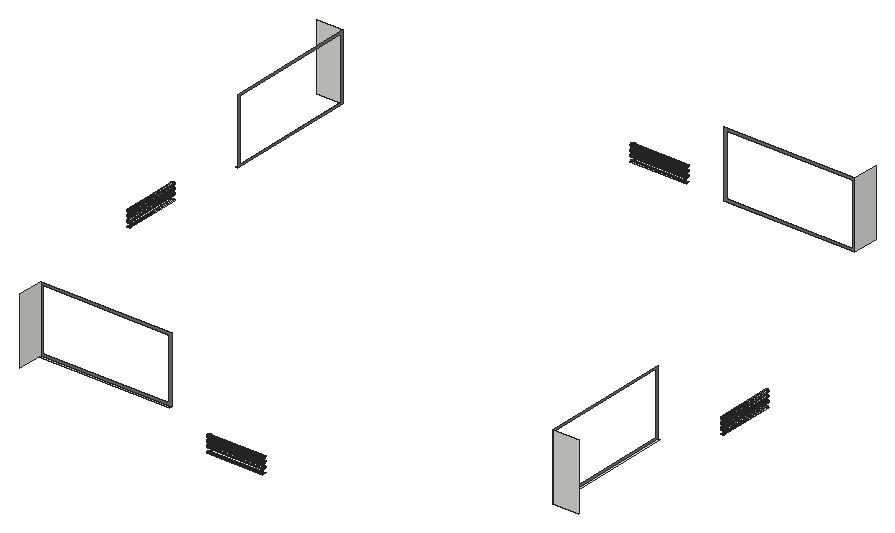
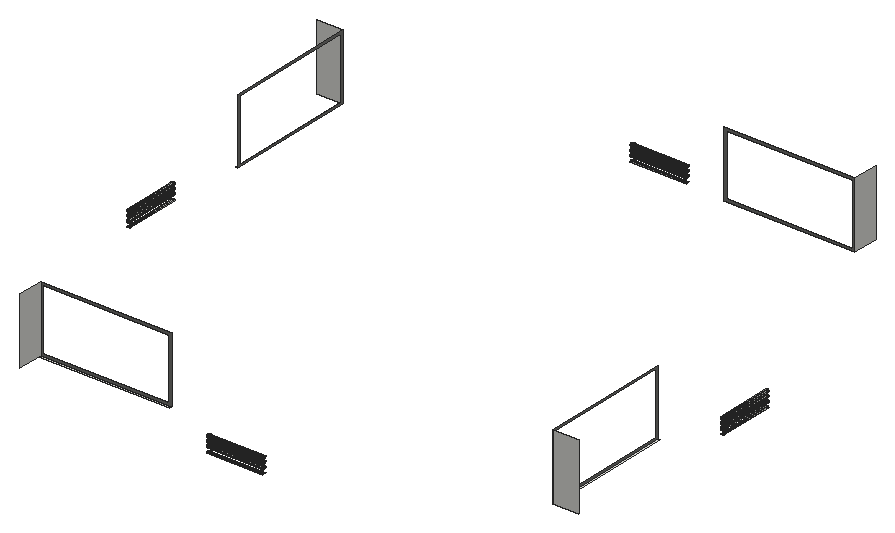
# SketchUp Ruby script. Lengths in inches.
U = 1.inch
M = Sketchup.active_model
def pt(a) = Geom::Point3d.new(a.map { |v| v * U })
def face(e, loops, mat)
  f = e.add_face(loops[0].map { |a| pt(a) })
  loops[1..].each { |l| e.add_face(l.map { |a| pt(a) }).erase! }
  f.material = f.back_material = mat if mat
  f
end
# faces: each face lists its corners as indices into pts; further lists are holes
def faces(e, pts, list, mat = nil) = list.each { |f| face(e, (f[0].is_a?(Array) ? f : [f]).map { |l| l.map { |i| pts[i] } }, mat) }
# xy, xz, yz: faces in a plane at the given z, y or x. An outline is a flat list of corners, or four numbers for a rectangle; further outlines are holes
def ring(l) = l.size == 4 ? [[l[0], l[1]], [l[2], l[1]], [l[2], l[3]], [l[0], l[3]]] : l.each_slice(2).to_a
def flat(e, list, mat, &to3) = list.each { |f| face(e, (f[0].is_a?(Array) ? f : [f]).map { |l| ring(l).map { |u, v| to3.(u, v) } }, mat) }
def xy(e, z, list, mat = nil) = flat(e, list, mat) { |x, y| [x, y, z] }
def xz(e, y, list, mat = nil) = flat(e, list, mat) { |x, z| [x, y, z] }
def yz(e, x, list, mat = nil) = flat(e, list, mat) { |y, z| [x, y, z] }
def lines(e, pts, list) = list.each { |a, b| e.add_line(pt(pts[a]), pt(pts[b])) }
# prism: a flat outline (further loops are holes) pulled along v
def prism(e, loops, v, mat = nil)
  f = face(e, loops, mat); d = Geom::Vector3d.new(v.map { |x| x * U })
  f.pushpull(f.normal.samedirection?(d) ? d.length : -d.length)
end
def box(e, o, s, mat = nil) = prism(e, [[o, [o[0] + s[0], o[1], o[2]], [o[0] + s[0], o[1] + s[1], o[2]], [o[0], o[1] + s[1], o[2]]]], [0, 0, s[2]], mat)
def at(x, y, z, deg = 0) = Geom::Transformation.translation(pt([x, y, z])) * Geom::Transformation.rotation(ORIGIN, Z_AXIS, deg.degrees)
def axes(o, x, y, z) = Geom::Transformation.new([*x, 0, *y, 0, *z, 0, *pt(o).to_a, 1])
def part(name) = M.definitions.add(name)
# library, detail: a bought-in or finely detailed component or shape, given as its bounding box
def library(name, o, s) = part(name).tap { |d| box(d.entities, o, s) }
def detail(e, o, s) = box(e.add_group.entities, o, s)
def put(e, d, t, mat = nil) = e.add_instance(d, t).tap { |i| i.material = mat if mat }
def group(e, t, mat = nil) = e.add_group.tap { |g| g.transformation = t; g.material = mat if mat }.entities
root = M.entities
M.materials.add("[Metal Seamed]").color = [118, 119, 115]
xy(root,533.76,[[306.65,96.8125,641.22,102.8125],[1482,271.47,1488,606.03],[132,943.59,138,1278.16],[978.78,1446.8125,1313.35,1452.8125]])
xz(root,102.8125,[[[306.65,533.76,641.22,702.625],[312.65,539.76,635.22,696.625]]],"[Metal Seamed]")
xz(root,271.47,[[1482,533.76,1548,702.625]])
xz(root,1278.16,[[72,533.76,138,702.625]])
xz(root,1446.8125,[[[978.78,533.76,1313.35,702.625],[984.78,539.76,1307.35,696.625]]],"[Metal Seamed]")
yz(root,138,[[[943.59,533.76,1278.16,702.625],[949.59,539.76,1272.16,696.625]]],"[Metal Seamed]")
yz(root,306.65,[[36.8125,533.76,102.8125,702.625]])
yz(root,1313.35,[[1446.8125,533.76,1512.8125,702.625]])
yz(root,1482,[[[271.47,533.76,606.03,702.625],[277.47,539.76,600.03,696.625]]],"[Metal Seamed]")
p = [[922.01,44.78,502.66],[922.01,45.15,503.55],[778.64,45.15,503.55],[778.64,44.78,502.66],[922.01,51.53,503.55],[922.01,51.9,502.66],
  [778.64,51.9,502.66],[778.64,51.53,503.55],[79.97,662.8,502.66],[80.33,662.8,503.55],[80.33,806.17,503.55],[79.97,806.17,502.66],
  [86.72,662.8,503.55],[87.09,662.8,502.66],[87.09,806.17,502.66],[86.72,806.17,503.55],[1533.28,886.83,503.55],[1532.91,886.83,502.66],
  [1532.91,743.45,502.66],[1533.28,743.45,503.55],[1540.03,886.83,502.66],[1539.67,886.83,503.55],[1539.67,743.45,503.55],[1540.03,743.45,502.66],
  [697.99,1498.09,503.55],[697.99,1497.72,502.66],[841.36,1497.72,502.66],[841.36,1498.09,503.55],[697.99,1504.85,502.66],[697.99,1504.48,503.55],
  [841.36,1504.48,503.55],[841.36,1504.85,502.66],[922.01,45.73,504.3125],[778.64,45.73,504.3125],[922.01,50.95,504.3125],[778.64,50.95,504.3125],
  [80.92,662.8,504.3125],[80.92,806.17,504.3125],[86.13,662.8,504.3125],[86.13,806.17,504.3125],[1533.87,886.83,504.3125],[1533.87,743.45,504.3125],
  [1539.08,886.83,504.3125],[1539.08,743.45,504.3125],[697.99,1498.68,504.3125],[841.36,1498.68,504.3125],[697.99,1503.89,504.3125],[841.36,1503.89,504.3125],
  [922.01,46.5,504.9],[778.64,46.5,504.9],[922.01,50.18,504.9],[778.64,50.18,504.9],[81.68,662.8,504.9],[81.68,806.17,504.9],
  [85.37,662.8,504.9],[85.37,806.17,504.9],[1534.63,886.83,504.9],[1534.63,743.45,504.9],[1538.32,886.83,504.9],[1538.32,743.45,504.9],
  [697.99,1499.44,504.9],[841.36,1499.44,504.9],[697.99,1503.13,504.9],[841.36,1503.13,504.9],[922.01,47.38,505.27],[778.64,47.38,505.27],
  [922.01,49.29,505.27],[778.64,49.29,505.27],[82.57,662.8,505.27],[82.57,806.17,505.27],[84.48,662.8,505.27],[84.48,806.17,505.27],
  [1535.52,886.83,505.27],[1535.52,743.45,505.27],[1537.43,886.83,505.27],[1537.43,743.45,505.27],[697.99,1500.33,505.27],[841.36,1500.33,505.27],
  [697.99,1502.24,505.27],[841.36,1502.24,505.27],[922.01,48.34,505.39],[778.64,48.34,505.39],[83.53,662.8,505.39],[83.53,806.17,505.39],
  [1536.47,886.83,505.39],[1536.47,743.45,505.39],[697.99,1501.28,505.39],[841.36,1501.28,505.39],[922.01,48.34,513.02],[922.01,47.38,513.14],
  [778.64,47.38,513.14],[778.64,48.34,513.02],[922.01,49.29,513.14],[778.64,49.29,513.14],[83.53,662.8,513.02],[82.57,662.8,513.14],
  [82.57,806.17,513.14],[83.53,806.17,513.02],[84.48,662.8,513.14],[84.48,806.17,513.14],[1535.52,886.83,513.14],[1536.47,886.83,513.02],
  [1536.47,743.45,513.02],[1535.52,743.45,513.14],[1537.43,886.83,513.14],[1537.43,743.45,513.14],[697.99,1500.33,513.14],[697.99,1501.28,513.02],
  [841.36,1501.28,513.02],[841.36,1500.33,513.14],[697.99,1502.24,513.14],[841.36,1502.24,513.14],[922.01,46.5,513.51],[778.64,46.5,513.51],
  [922.01,50.18,513.51],[778.64,50.18,513.51],[81.68,662.8,513.51],[81.68,806.17,513.51],[85.37,662.8,513.51],[85.37,806.17,513.51],
  [1534.63,886.83,513.51],[1534.63,743.45,513.51],[1538.32,886.83,513.51],[1538.32,743.45,513.51],[697.99,1499.44,513.51],[841.36,1499.44,513.51],
  [697.99,1503.13,513.51],[841.36,1503.13,513.51],[922.01,45.73,514.1],[778.64,45.73,514.1],[922.01,50.95,514.1],[778.64,50.95,514.1],
  [80.92,662.8,514.1],[80.92,806.17,514.1],[86.13,662.8,514.1],[86.13,806.17,514.1],[1533.87,886.83,514.1],[1533.87,743.45,514.1],
  [1539.08,886.83,514.1],[1539.08,743.45,514.1],[697.99,1498.68,514.1],[841.36,1498.68,514.1],[697.99,1503.89,514.1],[841.36,1503.89,514.1],
  [922.01,45.15,514.86],[778.64,45.15,514.86],[922.01,51.53,514.86],[778.64,51.53,514.86],[80.33,662.8,514.86],[80.33,806.17,514.86],
  [86.72,662.8,514.86],[86.72,806.17,514.86],[1533.28,886.83,514.86],[1533.28,743.45,514.86],[1539.67,886.83,514.86],[1539.67,743.45,514.86],
  [697.99,1498.09,514.86],[841.36,1498.09,514.86],[697.99,1504.48,514.86],[841.36,1504.48,514.86],[922.01,44.78,515.75],[778.64,44.78,515.75],
  [922.01,51.9,515.75],[778.64,51.9,515.75],[79.97,662.8,515.75],[79.97,806.17,515.75],[87.09,662.8,515.75],[87.09,806.17,515.75],
  [1532.91,886.83,515.75],[1532.91,743.45,515.75],[1540.03,886.83,515.75],[1540.03,743.45,515.75],[697.99,1497.72,515.75],[841.36,1497.72,515.75],
  [697.99,1504.85,515.75],[841.36,1504.85,515.75],[922.01,44.65,516.7],[778.64,44.65,516.7],[922.01,52.03,516.7],[778.64,52.03,516.7],
  [79.84,662.8,516.7],[79.84,806.17,516.7],[87.21,662.8,516.7],[87.21,806.17,516.7],[1532.79,886.83,516.7],[1532.79,743.45,516.7],
  [1540.16,886.83,516.7],[1540.16,743.45,516.7],[697.99,1497.6,516.7],[841.36,1497.6,516.7],[697.99,1504.97,516.7],[841.36,1504.97,516.7],
  [922.01,44.78,517.66],[778.64,44.78,517.66],[922.01,51.9,517.66],[778.64,51.9,517.66],[79.97,662.8,517.66],[79.97,806.17,517.66],
  [87.09,662.8,517.66],[87.09,806.17,517.66],[1532.91,886.83,517.66],[1532.91,743.45,517.66],[1540.03,886.83,517.66],[1540.03,743.45,517.66],
  [697.99,1497.72,517.66],[841.36,1497.72,517.66],[697.99,1504.85,517.66],[841.36,1504.85,517.66],[922.01,45.15,518.55],[778.64,45.15,518.55],
  [922.01,51.53,518.55],[778.64,51.53,518.55],[80.33,662.8,518.55],[80.33,806.17,518.55],[86.72,662.8,518.55],[86.72,806.17,518.55],
  [1533.28,886.83,518.55],[1533.28,743.45,518.55],[1539.67,886.83,518.55],[1539.67,743.45,518.55],[697.99,1498.09,518.55],[841.36,1498.09,518.55],
  [697.99,1504.48,518.55],[841.36,1504.48,518.55],[922.01,45.73,519.3125],[778.64,45.73,519.3125],[922.01,50.95,519.3125],[778.64,50.95,519.3125],
  [80.92,662.8,519.3125],[80.92,806.17,519.3125],[86.13,662.8,519.3125],[86.13,806.17,519.3125],[1533.87,886.83,519.3125],[1533.87,743.45,519.3125],
  [1539.08,886.83,519.3125],[1539.08,743.45,519.3125],[697.99,1498.68,519.3125],[841.36,1498.68,519.3125],[697.99,1503.89,519.3125],[841.36,1503.89,519.3125],
  [922.01,46.5,519.9],[778.64,46.5,519.9],[922.01,50.18,519.9],[778.64,50.18,519.9],[81.68,662.8,519.9],[81.68,806.17,519.9],
  [85.37,662.8,519.9],[85.37,806.17,519.9],[1534.63,886.83,519.9],[1534.63,743.45,519.9],[1538.32,886.83,519.9],[1538.32,743.45,519.9],
  [697.99,1499.44,519.9],[841.36,1499.44,519.9],[697.99,1503.13,519.9],[841.36,1503.13,519.9],[922.01,47.38,520.27],[778.64,47.38,520.27],
  [922.01,49.29,520.27],[778.64,49.29,520.27],[82.57,662.8,520.27],[82.57,806.17,520.27],[84.48,662.8,520.27],[84.48,806.17,520.27],
  [1535.52,886.83,520.27],[1535.52,743.45,520.27],[1537.43,886.83,520.27],[1537.43,743.45,520.27],[697.99,1500.33,520.27],[841.36,1500.33,520.27],
  [697.99,1502.24,520.27],[841.36,1502.24,520.27],[922.01,48.34,520.39],[778.64,48.34,520.39],[83.53,662.8,520.39],[83.53,806.17,520.39],
  [1536.47,886.83,520.39],[1536.47,743.45,520.39],[697.99,1501.28,520.39],[841.36,1501.28,520.39],[922.01,48.34,525.02],[922.01,47.38,525.14],
  [778.64,47.38,525.14],[778.64,48.34,525.02],[922.01,49.29,525.14],[778.64,49.29,525.14],[83.53,662.8,525.02],[82.57,662.8,525.14],
  [82.57,806.17,525.14],[83.53,806.17,525.02],[84.48,662.8,525.14],[84.48,806.17,525.14],[1535.52,886.83,525.14],[1536.47,886.83,525.02],
  [1536.47,743.45,525.02],[1535.52,743.45,525.14],[1537.43,886.83,525.14],[1537.43,743.45,525.14],[697.99,1500.33,525.14],[697.99,1501.28,525.02],
  [841.36,1501.28,525.02],[841.36,1500.33,525.14],[697.99,1502.24,525.14],[841.36,1502.24,525.14],[922.01,46.5,525.51],[778.64,46.5,525.51],
  [922.01,50.18,525.51],[778.64,50.18,525.51],[81.68,662.8,525.51],[81.68,806.17,525.51],[85.37,662.8,525.51],[85.37,806.17,525.51],
  [1534.63,886.83,525.51],[1534.63,743.45,525.51],[1538.32,886.83,525.51],[1538.32,743.45,525.51],[697.99,1499.44,525.51],[841.36,1499.44,525.51],
  [697.99,1503.13,525.51],[841.36,1503.13,525.51],[922.01,45.73,526.1],[778.64,45.73,526.1],[922.01,50.95,526.1],[778.64,50.95,526.1],
  [80.92,662.8,526.1],[80.92,806.17,526.1],[86.13,662.8,526.1],[86.13,806.17,526.1],[1533.87,886.83,526.1],[1533.87,743.45,526.1],
  [1539.08,886.83,526.1],[1539.08,743.45,526.1],[697.99,1498.68,526.1],[841.36,1498.68,526.1],[697.99,1503.89,526.1],[841.36,1503.89,526.1],
  [922.01,45.15,526.86],[778.64,45.15,526.86],[922.01,51.53,526.86],[778.64,51.53,526.86],[80.33,662.8,526.86],[80.33,806.17,526.86],
  [86.72,662.8,526.86],[86.72,806.17,526.86],[1533.28,886.83,526.86],[1533.28,743.45,526.86],[1539.67,886.83,526.86],[1539.67,743.45,526.86],
  [697.99,1498.09,526.86],[841.36,1498.09,526.86],[697.99,1504.48,526.86],[841.36,1504.48,526.86],[922.01,44.78,527.75],[778.64,44.78,527.75],
  [922.01,51.9,527.75],[778.64,51.9,527.75],[79.97,662.8,527.75],[79.97,806.17,527.75],[87.09,662.8,527.75],[87.09,806.17,527.75],
  [1532.91,886.83,527.75],[1532.91,743.45,527.75],[1540.03,886.83,527.75],[1540.03,743.45,527.75],[697.99,1497.72,527.75],[841.36,1497.72,527.75],
  [697.99,1504.85,527.75],[841.36,1504.85,527.75],[922.01,44.65,528.7],[778.64,44.65,528.7],[922.01,52.03,528.7],[778.64,52.03,528.7],
  [79.84,662.8,528.7],[79.84,806.17,528.7],[87.21,662.8,528.7],[87.21,806.17,528.7],[1532.79,886.83,528.7],[1532.79,743.45,528.7],
  [1540.16,886.83,528.7],[1540.16,743.45,528.7],[697.99,1497.6,528.7],[841.36,1497.6,528.7],[697.99,1504.97,528.7],[841.36,1504.97,528.7],
  [922.01,44.78,529.66],[778.64,44.78,529.66],[922.01,51.9,529.66],[778.64,51.9,529.66],[79.97,662.8,529.66],[79.97,806.17,529.66],
  [87.09,662.8,529.66],[87.09,806.17,529.66],[1532.91,886.83,529.66],[1532.91,743.45,529.66],[1540.03,886.83,529.66],[1540.03,743.45,529.66],
  [697.99,1497.72,529.66],[841.36,1497.72,529.66],[697.99,1504.85,529.66],[841.36,1504.85,529.66],[922.01,45.15,530.55],[778.64,45.15,530.55],
  [922.01,51.53,530.55],[778.64,51.53,530.55],[80.33,662.8,530.55],[80.33,806.17,530.55],[86.72,662.8,530.55],[86.72,806.17,530.55],
  [1533.28,886.83,530.55],[1533.28,743.45,530.55],[1539.67,886.83,530.55],[1539.67,743.45,530.55],[697.99,1498.09,530.55],[841.36,1498.09,530.55],
  [697.99,1504.48,530.55],[841.36,1504.48,530.55],[922.01,45.73,531.3125],[778.64,45.73,531.3125],[922.01,50.95,531.3125],[778.64,50.95,531.3125],
  [80.92,662.8,531.3125],[80.92,806.17,531.3125],[86.13,662.8,531.3125],[86.13,806.17,531.3125],[1533.87,886.83,531.3125],[1533.87,743.45,531.3125],
  [1539.08,886.83,531.3125],[1539.08,743.45,531.3125],[697.99,1498.68,531.3125],[841.36,1498.68,531.3125],[697.99,1503.89,531.3125],[841.36,1503.89,531.3125],
  [922.01,46.5,531.9],[778.64,46.5,531.9],[922.01,50.18,531.9],[778.64,50.18,531.9],[81.68,662.8,531.9],[81.68,806.17,531.9],
  [85.37,662.8,531.9],[85.37,806.17,531.9],[1534.63,886.83,531.9],[1534.63,743.45,531.9],[1538.32,886.83,531.9],[1538.32,743.45,531.9],
  [697.99,1499.44,531.9],[841.36,1499.44,531.9],[697.99,1503.13,531.9],[841.36,1503.13,531.9],[922.01,47.38,532.27],[778.64,47.38,532.27],
  [922.01,49.29,532.27],[778.64,49.29,532.27],[82.57,662.8,532.27],[82.57,806.17,532.27],[84.48,662.8,532.27],[84.48,806.17,532.27],
  [1535.52,886.83,532.27],[1535.52,743.45,532.27],[1537.43,886.83,532.27],[1537.43,743.45,532.27],[697.99,1500.33,532.27],[841.36,1500.33,532.27],
  [697.99,1502.24,532.27],[841.36,1502.24,532.27],[922.01,48.34,532.39],[778.64,48.34,532.39],[83.53,662.8,532.39],[83.53,806.17,532.39],
  [1536.47,886.83,532.39],[1536.47,743.45,532.39],[697.99,1501.28,532.39],[841.36,1501.28,532.39],[922.01,48.34,537.02],[922.01,47.38,537.14],
  [778.64,47.38,537.14],[778.64,48.34,537.02],[922.01,49.29,537.14],[778.64,49.29,537.14],[83.53,662.8,537.02],[82.57,662.8,537.14],
  [82.57,806.17,537.14],[83.53,806.17,537.02],[84.48,662.8,537.14],[84.48,806.17,537.14],[1535.52,886.83,537.14],[1536.47,886.83,537.02],
  [1536.47,743.45,537.02],[1535.52,743.45,537.14],[1537.43,886.83,537.14],[1537.43,743.45,537.14],[697.99,1500.33,537.14],[697.99,1501.28,537.02],
  [841.36,1501.28,537.02],[841.36,1500.33,537.14],[697.99,1502.24,537.14],[841.36,1502.24,537.14],[922.01,46.5,537.51],[778.64,46.5,537.51],
  [922.01,50.18,537.51],[778.64,50.18,537.51],[81.68,662.8,537.51],[81.68,806.17,537.51],[85.37,662.8,537.51],[85.37,806.17,537.51],
  [1534.63,886.83,537.51],[1534.63,743.45,537.51],[1538.32,886.83,537.51],[1538.32,743.45,537.51],[697.99,1499.44,537.51],[841.36,1499.44,537.51],
  [697.99,1503.13,537.51],[841.36,1503.13,537.51],[922.01,45.73,538.1],[778.64,45.73,538.1],[922.01,50.95,538.1],[778.64,50.95,538.1],
  [80.92,662.8,538.1],[80.92,806.17,538.1],[86.13,662.8,538.1],[86.13,806.17,538.1],[1533.87,886.83,538.1],[1533.87,743.45,538.1],
  [1539.08,886.83,538.1],[1539.08,743.45,538.1],[697.99,1498.68,538.1],[841.36,1498.68,538.1],[697.99,1503.89,538.1],[841.36,1503.89,538.1],
  [922.01,45.15,538.86],[778.64,45.15,538.86],[922.01,51.53,538.86],[778.64,51.53,538.86],[80.33,662.8,538.86],[80.33,806.17,538.86],
  [86.72,662.8,538.86],[86.72,806.17,538.86],[1533.28,886.83,538.86],[1533.28,743.45,538.86],[1539.67,886.83,538.86],[1539.67,743.45,538.86],
  [697.99,1498.09,538.86],[841.36,1498.09,538.86],[697.99,1504.48,538.86],[841.36,1504.48,538.86],[922.01,44.78,539.75],[778.64,44.78,539.75],
  [922.01,51.9,539.75],[778.64,51.9,539.75],[79.97,662.8,539.75],[79.97,806.17,539.75],[87.09,662.8,539.75],[87.09,806.17,539.75],
  [1532.91,886.83,539.75],[1532.91,743.45,539.75],[1540.03,886.83,539.75],[1540.03,743.45,539.75],[697.99,1497.72,539.75],[841.36,1497.72,539.75],
  [697.99,1504.85,539.75],[841.36,1504.85,539.75],[922.01,44.65,540.7],[778.64,44.65,540.7],[922.01,52.03,540.7],[778.64,52.03,540.7],
  [79.84,662.8,540.7],[79.84,806.17,540.7],[87.21,662.8,540.7],[87.21,806.17,540.7],[1532.79,886.83,540.7],[1532.79,743.45,540.7],
  [1540.16,886.83,540.7],[1540.16,743.45,540.7],[697.99,1497.6,540.7],[841.36,1497.6,540.7],[697.99,1504.97,540.7],[841.36,1504.97,540.7],
  [922.01,44.78,541.66],[778.64,44.78,541.66],[922.01,51.9,541.66],[778.64,51.9,541.66],[79.97,662.8,541.66],[79.97,806.17,541.66],
  [87.09,662.8,541.66],[87.09,806.17,541.66],[1532.91,886.83,541.66],[1532.91,743.45,541.66],[1540.03,886.83,541.66],[1540.03,743.45,541.66],
  [697.99,1497.72,541.66],[841.36,1497.72,541.66],[697.99,1504.85,541.66],[841.36,1504.85,541.66],[922.01,45.15,542.55],[778.64,45.15,542.55],
  [922.01,51.53,542.55],[778.64,51.53,542.55],[80.33,662.8,542.55],[80.33,806.17,542.55],[86.72,662.8,542.55],[86.72,806.17,542.55],
  [1533.28,886.83,542.55],[1533.28,743.45,542.55],[1539.67,886.83,542.55],[1539.67,743.45,542.55],[697.99,1498.09,542.55],[841.36,1498.09,542.55],
  [697.99,1504.48,542.55],[841.36,1504.48,542.55],[922.01,45.73,543.3125],[778.64,45.73,543.3125],[922.01,50.95,543.3125],[778.64,50.95,543.3125],
  [80.92,662.8,543.3125],[80.92,806.17,543.3125],[86.13,662.8,543.3125],[86.13,806.17,543.3125],[1533.87,886.83,543.3125],[1533.87,743.45,543.3125],
  [1539.08,886.83,543.3125],[1539.08,743.45,543.3125],[697.99,1498.68,543.3125],[841.36,1498.68,543.3125],[697.99,1503.89,543.3125],[841.36,1503.89,543.3125],
  [922.01,46.5,543.9],[778.64,46.5,543.9],[922.01,50.18,543.9],[778.64,50.18,543.9],[81.68,662.8,543.9],[81.68,806.17,543.9],
  [85.37,662.8,543.9],[85.37,806.17,543.9],[1534.63,886.83,543.9],[1534.63,743.45,543.9],[1538.32,886.83,543.9],[1538.32,743.45,543.9],
  [697.99,1499.44,543.9],[841.36,1499.44,543.9],[697.99,1503.13,543.9],[841.36,1503.13,543.9],[922.01,47.38,544.27],[778.64,47.38,544.27],
  [922.01,49.29,544.27],[778.64,49.29,544.27],[82.57,662.8,544.27],[82.57,806.17,544.27],[84.48,662.8,544.27],[84.48,806.17,544.27],
  [1535.52,886.83,544.27],[1535.52,743.45,544.27],[1537.43,886.83,544.27],[1537.43,743.45,544.27],[697.99,1500.33,544.27],[841.36,1500.33,544.27],
  [697.99,1502.24,544.27],[841.36,1502.24,544.27],[922.01,48.34,544.39],[778.64,48.34,544.39],[83.53,662.8,544.39],[83.53,806.17,544.39],
  [1536.47,886.83,544.39],[1536.47,743.45,544.39],[697.99,1501.28,544.39],[841.36,1501.28,544.39]]
faces(root,p,[[0,1,2,3],[4,5,6,7],[8,9,10,11],[12,13,14,15],[16,17,18,19],[20,21,22,23],[24,25,26,27],[28,29,30,31],
  [1,32,33,2],[34,4,7,35],[9,36,37,10],[38,12,15,39],[40,16,19,41],[21,42,43,22],[44,24,27,45],[29,46,47,30],
  [32,48,49,33],[50,34,35,51],[36,52,53,37],[54,38,39,55],[56,40,41,57],[42,58,59,43],[60,44,45,61],[46,62,63,47],
  [48,64,65,49],[66,50,51,67],[52,68,69,53],[70,54,55,71],[72,56,57,73],[58,74,75,59],[76,60,61,77],[62,78,79,63],
  [64,80,81,65],[80,66,67,81],[68,82,83,69],[82,70,71,83],[84,72,73,85],[74,84,85,75],[86,76,77,87],[78,86,87,79],
  [88,89,90,91],[92,88,91,93],[94,95,96,97],[98,94,97,99],[100,101,102,103],[101,104,105,102],[106,107,108,109],[107,110,111,108],
  [89,112,113,90],[114,92,93,115],[95,116,117,96],[118,98,99,119],[120,100,103,121],[104,122,123,105],[124,106,109,125],[110,126,127,111],
  [112,128,129,113],[130,114,115,131],[116,132,133,117],[134,118,119,135],[136,120,121,137],[122,138,139,123],[140,124,125,141],[126,142,143,127],
  [128,144,145,129],[146,130,131,147],[132,148,149,133],[150,134,135,151],[152,136,137,153],[138,154,155,139],[156,140,141,157],[142,158,159,143],
  [144,160,161,145],[162,146,147,163],[148,164,165,149],[166,150,151,167],[168,152,153,169],[154,170,171,155],[172,156,157,173],[158,174,175,159],
  [160,176,177,161],[178,162,163,179],[164,180,181,165],[182,166,167,183],[184,168,169,185],[170,186,187,171],[188,172,173,189],[174,190,191,175],
  [176,192,193,177],[194,178,179,195],[180,196,197,181],[198,182,183,199],[200,184,185,201],[186,202,203,187],[204,188,189,205],[190,206,207,191],
  [192,208,209,193],[210,194,195,211],[196,212,213,197],[214,198,199,215],[216,200,201,217],[202,218,219,203],[220,204,205,221],[206,222,223,207],
  [208,224,225,209],[226,210,211,227],[212,228,229,213],[230,214,215,231],[232,216,217,233],[218,234,235,219],[236,220,221,237],[222,238,239,223],
  [224,240,241,225],[242,226,227,243],[228,244,245,229],[246,230,231,247],[248,232,233,249],[234,250,251,235],[252,236,237,253],[238,254,255,239],
  [240,256,257,241],[258,242,243,259],[244,260,261,245],[262,246,247,263],[264,248,249,265],[250,266,267,251],[268,252,253,269],[254,270,271,255],
  [256,272,273,257],[272,258,259,273],[260,274,275,261],[274,262,263,275],[276,264,265,277],[266,276,277,267],[278,268,269,279],[270,278,279,271],
  [280,281,282,283],[284,280,283,285],[286,287,288,289],[290,286,289,291],[292,293,294,295],[293,296,297,294],[298,299,300,301],[299,302,303,300],
  [281,304,305,282],[306,284,285,307],[287,308,309,288],[310,290,291,311],[312,292,295,313],[296,314,315,297],[316,298,301,317],[302,318,319,303],
  [304,320,321,305],[322,306,307,323],[308,324,325,309],[326,310,311,327],[328,312,313,329],[314,330,331,315],[332,316,317,333],[318,334,335,319],
  [320,336,337,321],[338,322,323,339],[324,340,341,325],[342,326,327,343],[344,328,329,345],[330,346,347,331],[348,332,333,349],[334,350,351,335],
  [336,352,353,337],[354,338,339,355],[340,356,357,341],[358,342,343,359],[360,344,345,361],[346,362,363,347],[364,348,349,365],[350,366,367,351],
  [352,368,369,353],[370,354,355,371],[356,372,373,357],[374,358,359,375],[376,360,361,377],[362,378,379,363],[380,364,365,381],[366,382,383,367],
  [368,384,385,369],[386,370,371,387],[372,388,389,373],[390,374,375,391],[392,376,377,393],[378,394,395,379],[396,380,381,397],[382,398,399,383],
  [384,400,401,385],[402,386,387,403],[388,404,405,389],[406,390,391,407],[408,392,393,409],[394,410,411,395],[412,396,397,413],[398,414,415,399],
  [400,416,417,401],[418,402,403,419],[404,420,421,405],[422,406,407,423],[424,408,409,425],[410,426,427,411],[428,412,413,429],[414,430,431,415],
  [416,432,433,417],[434,418,419,435],[420,436,437,421],[438,422,423,439],[440,424,425,441],[426,442,443,427],[444,428,429,445],[430,446,447,431],
  [432,448,449,433],[450,434,435,451],[436,452,453,437],[454,438,439,455],[456,440,441,457],[442,458,459,443],[460,444,445,461],[446,462,463,447],
  [448,464,465,449],[464,450,451,465],[452,466,467,453],[466,454,455,467],[468,456,457,469],[458,468,469,459],[470,460,461,471],[462,470,471,463],
  [472,473,474,475],[476,472,475,477],[478,479,480,481],[482,478,481,483],[484,485,486,487],[485,488,489,486],[490,491,492,493],[491,494,495,492],
  [473,496,497,474],[498,476,477,499],[479,500,501,480],[502,482,483,503],[504,484,487,505],[488,506,507,489],[508,490,493,509],[494,510,511,495],
  [496,512,513,497],[514,498,499,515],[500,516,517,501],[518,502,503,519],[520,504,505,521],[506,522,523,507],[524,508,509,525],[510,526,527,511],
  [512,528,529,513],[530,514,515,531],[516,532,533,517],[534,518,519,535],[536,520,521,537],[522,538,539,523],[540,524,525,541],[526,542,543,527],
  [528,544,545,529],[546,530,531,547],[532,548,549,533],[550,534,535,551],[552,536,537,553],[538,554,555,539],[556,540,541,557],[542,558,559,543],
  [544,560,561,545],[562,546,547,563],[548,564,565,549],[566,550,551,567],[568,552,553,569],[554,570,571,555],[572,556,557,573],[558,574,575,559],
  [560,576,577,561],[578,562,563,579],[564,580,581,565],[582,566,567,583],[584,568,569,585],[570,586,587,571],[588,572,573,589],[574,590,591,575],
  [576,592,593,577],[594,578,579,595],[580,596,597,581],[598,582,583,599],[600,584,585,601],[586,602,603,587],[604,588,589,605],[590,606,607,591],
  [592,608,609,593],[610,594,595,611],[596,612,613,597],[614,598,599,615],[616,600,601,617],[602,618,619,603],[620,604,605,621],[606,622,623,607],
  [608,624,625,609],[626,610,611,627],[612,628,629,613],[630,614,615,631],[632,616,617,633],[618,634,635,619],[636,620,621,637],[622,638,639,623],
  [624,640,641,625],[642,626,627,643],[628,644,645,629],[646,630,631,647],[648,632,633,649],[634,650,651,635],[652,636,637,653],[638,654,655,639],
  [640,656,657,641],[656,642,643,657],[644,658,659,645],[658,646,647,659],[660,648,649,661],[650,660,661,651],[662,652,653,663],[654,662,663,655]])
